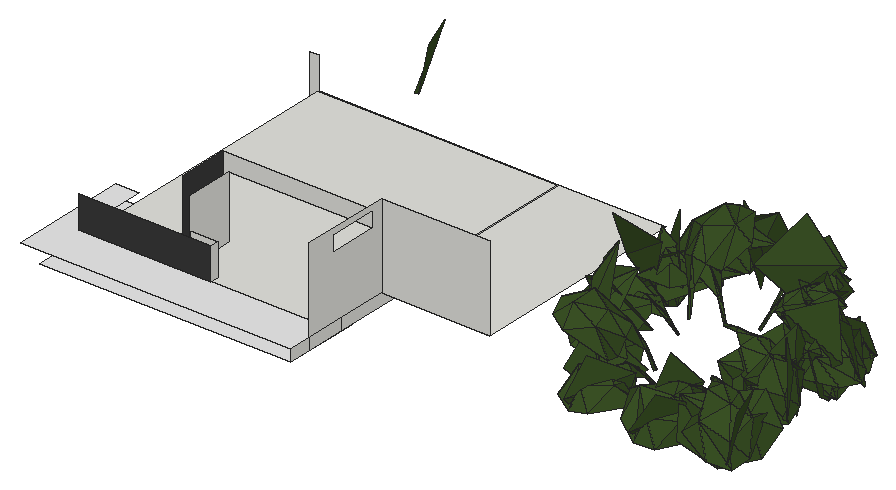
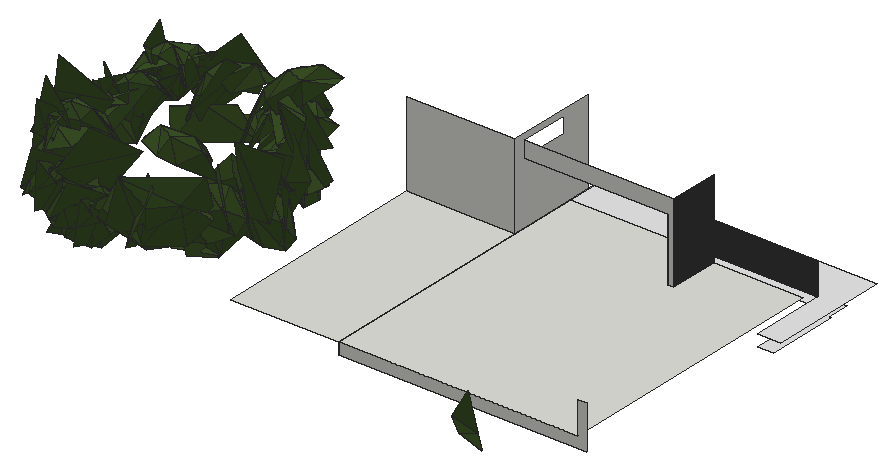
# SketchUp Ruby script. Lengths in inches.
U = 1.inch
M = Sketchup.active_model
def pt(a) = Geom::Point3d.new(a.map { |v| v * U })
def face(e, loops, mat)
  f = e.add_face(loops[0].map { |a| pt(a) })
  loops[1..].each { |l| e.add_face(l.map { |a| pt(a) }).erase! }
  f.material = f.back_material = mat if mat
  f
end
# faces: each face lists its corners as indices into pts; further lists are holes
def faces(e, pts, list, mat = nil) = list.each { |f| face(e, (f[0].is_a?(Array) ? f : [f]).map { |l| l.map { |i| pts[i] } }, mat) }
# xy, xz, yz: faces in a plane at the given z, y or x. An outline is a flat list of corners, or four numbers for a rectangle; further outlines are holes
def ring(l) = l.size == 4 ? [[l[0], l[1]], [l[2], l[1]], [l[2], l[3]], [l[0], l[3]]] : l.each_slice(2).to_a
def flat(e, list, mat, &to3) = list.each { |f| face(e, (f[0].is_a?(Array) ? f : [f]).map { |l| ring(l).map { |u, v| to3.(u, v) } }, mat) }
def xy(e, z, list, mat = nil) = flat(e, list, mat) { |x, y| [x, y, z] }
def xz(e, y, list, mat = nil) = flat(e, list, mat) { |x, z| [x, y, z] }
def yz(e, x, list, mat = nil) = flat(e, list, mat) { |y, z| [x, y, z] }
def lines(e, pts, list) = list.each { |a, b| e.add_line(pt(pts[a]), pt(pts[b])) }
# prism: a flat outline (further loops are holes) pulled along v
def prism(e, loops, v, mat = nil)
  f = face(e, loops, mat); d = Geom::Vector3d.new(v.map { |x| x * U })
  f.pushpull(f.normal.samedirection?(d) ? d.length : -d.length)
end
def box(e, o, s, mat = nil) = prism(e, [[o, [o[0] + s[0], o[1], o[2]], [o[0] + s[0], o[1] + s[1], o[2]], [o[0], o[1] + s[1], o[2]]]], [0, 0, s[2]], mat)
def at(x, y, z, deg = 0) = Geom::Transformation.translation(pt([x, y, z])) * Geom::Transformation.rotation(ORIGIN, Z_AXIS, deg.degrees)
def axes(o, x, y, z) = Geom::Transformation.new([*x, 0, *y, 0, *z, 0, *pt(o).to_a, 1])
def part(name) = M.definitions.add(name)
# library, detail: a bought-in or finely detailed component or shape, given as its bounding box
def library(name, o, s) = part(name).tap { |d| box(d.entities, o, s) }
def detail(e, o, s) = box(e.add_group.entities, o, s)
def put(e, d, t, mat = nil) = e.add_instance(d, t).tap { |i| i.material = mat if mat }
def group(e, t, mat = nil) = e.add_group.tap { |g| g.transformation = t; g.material = mat if mat }.entities
root = M.entities
M.materials.add("AM113_062_Tilia").color = [58, 81, 37]
M.materials.add("[Color M07]").color = [58, 58, 58]
M.materials.add("white_wall").color = [233, 233, 233]
xy(root,500.91,[[413.32,28.625,413.32,82.67,390.32,82.67,390.32,130.3125,385.62,130.3125,385.62,278.26,418.81,278.26,418.81,115.3125,496.21,115.3125,496.21,121.6875,695.48,121.6875,695.48,187.1875,935.92,187.1875,935.92,28.625]],"white_wall")
xy(root,525.1,[[695.48,121.6875,935.92,121.6875,935.92,725.65,436.99,725.65,436.99,139.5,622.42,139.5,622.42,242.3125,635.92,242.3125,635.92,139.5,695.48,139.5],[935.92,265.5,1160.625,725.65]])
xy(root,525.1,[[371.87,28.625,935.92,28.625,935.92,121.6875,418.81,121.6875,418.81,278.26,371.87,278.26]],"white_wall")
xz(root,121.6875,[[418.81,525.1,695.48,592.47]],"[Color M07]")
xz(root,139.5,[[635.92,525.1,695.48,592.47]])
xz(root,242.3125,[[622.42,525.1,622.42,690.29,935.92,690.29,935.92,656.55,635.92,656.55,635.92,525.1]])
xz(root,265.5,[[935.92,525.1,1160.625,701.22]])
xz(root,725.65,[[418.81,500.91,418.81,592.47,436.99,592.47,436.99,525.1,935.92,525.1,935.92,500.91]])
yz(root,622.42,[[139.5,525.1,242.3125,690.29]],"[Color M07]")
yz(root,635.92,[[139.5,525.1,242.3125,656.55]])
yz(root,695.48,[[121.6875,525.1,139.5,592.47]])
yz(root,935.92,[[28.625,500.91,76.875,525.1],[76.875,500.91,160.1875,525.1],[160.1875,500.91,725.65,525.1],[[76.875,525.1,265.5,701.22],[139.5,656.55,242.3125,690.29]]])
p = [[1608.53,201.41,601.09],[1641.49,153.68,545.55],[1685.26,205.85,485.78],[1680.28,206.99,573.08],[1711.38,254.78,570.88],[1727.03,267.14,493.375],
  [1227.45,504.22,507.09],[1257.77,498.2,487.25],[1308.93,432.76,542.29],[1230.67,494.24,489.34],[1237.69,460.03,493.43],[1244.5,488.78,535.27],
  [1286.74,524.49,559.43],[1250.26,531.08,507.09],[1301.88,581.08,490.56],[1299.69,508.34,521.98],[1300.21,541.42,597.74],[1294.36,601.5,579.96],
  [1342.6,650.07,597.52],[1301.32,663.28,529.03],[1620.96,549.03,509.56],[1665.6,554.86,490.94],[1667.41,568.21,523.57],[1682.46,602.0625,491.55],
  [1691.6,430.92,610.26],[1724.02,422.12,539.31],[1691.39,487.72,491.14],[1714.9375,485.36,573.8],[1691.59,538.34,581.77],[1672.27,556.16,507.36],
  [1668.61,633.98,501.61],[1337.11,293.34,491.66],[1387.67,242.25,499.89],[1388.19,266.96,575.1875],[1343.69,304.44,578.2],[1349.98,369.09,590.34],
  [1297.59,350.6,548.22],[1678.86,626.72,509.68],[1656.26,616.84,492.5],[1599.58,597.82,552.56],[1644.91,627.1875,572],[1630.5625,649.05,492.68],
  [1576.24,624.51,514.75],[1745.05,301.41,540.22],[1295.82,401.91,522.83],[1268.66,437.86,545.74],[1511.4,570.35,560.8],[1566.7,592.6875,494.25],
  [1616.57,617.13,543.95],[1503.48,634.35,576.94],[1520.24,677.18,494.31],[1535.15,738.46,525.68],[1599.58,313.53,611.65],[1643.34,292.87,542.47],
  [1654.98,365.88,495.65],[1658.99,353.22,581.5],[1666.94,409.27,590.46],[1667.95,437.21,517.2],[1711.86,395.82,596.52],[1685.69,410.02,495.72],
  [1631.72,447.7,548.77],[1657.73,307.26,600.03],[1661.35,300.36,517.51],[1635.08,376.57,496.53],[1681.1,359.02,557.6],[1677.27,414.18,581.15],
  [1641.67,444.67,526.12],[1453.5,335.59,497.8],[1443.43,306.41,535.73],[1449.4375,309.89,537.47],[1453.22,308.86,531.31],[1456.31,334.82,497.81],
  [1455.86,338.05,501.03],[1301.33,350.89,630.68],[1239.92,360.78,558.58],[1299.97,344.13,498.89],[1367.08,404.5,524.83],[1370.45,429.46,537.58],
  [1276.97,440.16,499.17],[1231.26,429.43,589.95],[1574,282.72,550.39],[1590.74,343.79,499.42],[1458.66,277.01,517.78],[1633.2,294.35,530.68],
  [1427.35,224.91,541.33],[1665.2,614.9375,533.37],[1645.59,642.78,519.97],[1372.92,271.21,623.86],[1333.62,243.31,535.71],[1406.36,250.31,501.97],
  [1433,337.17,524.2],[1543.93,687.91,601.39],[1560.58,714.84,549.01],[1506.53,704.21,502.82],[1508.01,717.95,570.93],[1449.125,701.42,508.87],
  [1462.29,709.39,571.11],[1279.84,345.16,502.99],[1312.67,305.26,522.83],[1304.35,350.98,578.03],[1258.94,412.12,524.86],[1635.5,421.94,588.94],
  [1701.53,411.0625,553.85],[1711.42,482.68,502.96],[1688.85,474.8,584.89],[1680.5,531.22,585.72],[1699.88,555.625,514.64],[1474.65,208.35,538.16],
  [1552.91,206.89,505.11],[1524.41,254.78,555.05],[1614.9375,247.95,507.18],[1286.14,594.98,505.61],[1274.16,520.22,535.21],[1314.23,544.61,597.49],
  [1325.53,603.12,582.9],[1396.83,635.1,561.15],[1329.75,667.15,536.15],[1314.83,358.71,573.32],[1300.05,304.08,539.93],[1359.23,329.29,505.88],
  [1352.78,470.5,565.37],[1301.03,422.38,570.82],[1237.73,477.64,588.08],[1306.48,546.06,533.875],[1662.44,591.39,558.45],[1668.39,175.84,581.64],
  [1696.45,159,523.32],[1731.08,184.67,508.39],[1722.59,190.66,557.13],[1741.22,217.9,518.5],[1417.19,697.9,545.89],[1662.07,319.36,582.11],
  [1688.34,324.3,518.9],[1707.34,363.98,509.22],[1702.21,359.18,558.95],[1703.72,396.45,527.51],[1729.71,172.23,524.3],[1704.85,194.06,509.27],
  [1691.77,269.78,580.98],[569.08,821.01,524.3],[544.22,842.83,509.27],[531.15,918.56,580.98],[1614.36,549.44,538.52],[1602.1,598.66,579.22],
  [1670.43,608.51,577.0625],[1573.15,571.08,602.63],[1611.93,580.5,560.65],[1576.44,619.48,510.05],[1576.88,620.47,580.45],[1536.41,660.93,512.41],
  [1541.04,649.93,575.9],[1720.67,530.4375,617.48],[1728.57,533.34,510.15],[1655.3,557.29,521.91],[1405.16,153.17,541.64],[1411.17,178.17,510.85],
  [1474.36,243.05,547.15],[1492.28,584.64,542.69],[1478.94,575.19,511.11],[1476.91,573.07,513],[1492.97,581.45,547.48],[1479.94,573.09,511.06],
  [1498.32,579.69,547.0625],[1507.43,679.5,545.82],[1322.69,293.23,514.1],[1367.74,234.48,523.55],[1395.16,278.09,571.02],[1363.4,325.46,570.48],
  [1383.97,392.54,535.68],[1315.3,371.51,545.73],[1712.89,350.28,521.46],[1679.92,360.82,514.2],[1644.1,412.73,605.58],[1680.69,590.25,560.28],
  [1513.4,718.2,514.57],[1510.84,695.24,577.86],[1541.9,643.84,579.47],[1564.26,694.65,559.0625],[1465.57,699.29,573.64],[1454.14,722.33,517.46],
  [1589.54,554.74,540.99],[1580.59,544.65,539.82],[1554.89,533.6,519.06],[1556.55,534.56,515.47],[1585.17,544.5,535.56],[1577.37,547.73,537.0625],
  [1555.3125,536.29,516.7],[1674.77,469.17,571.17],[1556.35,651.91,613.09],[1521.76,654.98,517.53],[1502.67,589.41,553.91],[1581.6875,663.6875,534.79],
  [1421.29,711.72,549.26],[1566.69,133.71,524.875],[1598.75,148.19,517.66],[1576.43,153.04,567.01],[1621.69,188.54,559.23],[1646.23,220.55,522.91],
  [1420.59,617.25,621.1],[1401.85,671.68,517.69],[1366.38,742.19,556.95],[1471.69,728.6875,602.9375],[1476.86,740.6,518.39],[1444.36,687.78,518.62],
  [1725.52,246.03,578.39],[1717.69,293.34,564.31],[1483.12,638.75,569.46],[1636.45,304.22,556.29],[1624.37,618.64,560.88],[1585.53,623.89,557.1],
  [1560.79,130.21,545.73],[1556.22,159.39,521.33],[1616.67,228.95,550.25],[1473.58,256.71,521.39],[1468.04,260.58,558.26],[1470.1,204.63,565.96],
  [1506.66,226.96,534.77],[1657.72,416.41,633.88],[1719.05,358.2,610.87],[1611.67,492.47,585.71],[1306.15,475.61,582.13],[1355.55,322.27,560.45],
  [1327.625,433.7,523.27],[1608.23,245.3,529.97],[1639.7,168.85,555.37],[1323.03,438.05,559.67],[1381.29,222.1,568.35],[1377.32,174.28,531.56],
  [1415.8,152.53,523.625],[1419.43,176.86,562.98],[1450.18,161.58,526.36],[1412.87,219.85,554.3],[1634.27,587.6,560],[1412.17,553.15,566.37],
  [1438.04,536.35,527.79],[1435.375,538.43,523.96],[1408.89,559.38,562.98],[1704.6,272.01,610.13],[1735.45,191.29,610.92],[543.97,920.79,610.13],
  [574.82,840.0625,610.92],[1536.19,189.6,597.59],[1529.56,147.08,551.74],[1284.17,401.26,605.55],[1321.77,452.63,626.16],[1261.18,466.59,604.29],
  [1410.2,548.1875,561.41],[1434.3125,535.63,525.01],[1499.07,721.84,601.54],[1542.79,546.8,567.91],[1597.85,563.92,564.49],[1589.35,621.96,526.02],
  [1560.88,603.25,580.4375],[1535.32,640.78,575.46],[1553.72,669.54,527.3125],[1658.55,474.5,579.81],[1519.73,684.8125,553.46],[1684.07,406.65,594.57],
  [1655.95,447.01,594.14],[1366.85,686.33,528.33],[1314.39,637.14,535.91],[1320.47,655.41,613.81],[1357.14,700.64,613.59],[1415.74,701.12,651.71],
  [1409.78,740.29,586.14],[1403.52,274,528.53],[1359.78,234.46,534.93],[1422.1,280.59,556.48],[1611.18,243.47,567.59],[1461.57,265.78,530.04],
  [1280.85,564.23,638.51],[1253.03,552.57,530.6],[1318.49,502.35,533.64],[1445.99,273.75,571.29],[1374.88,451.56,553.33],[1406.8,448.44,531.47],
  [1409.12,448.6875,535.73],[1263.05,341.63,531.83],[1250.26,413.28,551.72],[1557.84,196.35,585.28],[1554.79,207.85,542.72],[1564.06,301.86,531.88],
  [1566.56,316.89,559.1875],[1374.54,455.09,559.72],[1407.6,451.18,531.9],[1371.82,461.16,557.1],[1395.05,556.37,572.13],[1756.79,484.03,559.74],
  [1728.09,485.14,533.77],[1654.7,529.06,586.64],[1343.99,501.77,540.33],[1585.03,291.13,560.35],[1576.95,321.07,534.7],[1576.89,323.73,538.73],
  [1587.31,591.74,534.94],[1597.89,582.3,559.06],[1289.01,483.91,587.59],[1288.87,466.49,571.02],[1607.62,562.51,559.41],[1574.2,321.33,535.88],
  [1577.11,286.48,567.33],[1582.77,290.6875,567.76],[1286.8,607.89,582.24],[1449.44,311.51,578.55],[1455.06,326.86,535.96],[1457.43,329.96,537.64],
  [1479.73,626.03,562.03],[1477.46,604.47,536.34],[1477.82,601.97,539.04],[1482.75,625.38,567.01],[1479.71,603.87,536.36],[1487.54,628.14,565.49],
  [1453.36,329.1875,536.52],[1442.17,316,586.78],[1449.05,315.19,584.94],[1300.2,386.02,635.55],[1603.91,476.61,631.84],[1671.75,470.05,539.75],
  [1744.25,456.05,593.02],[1689.67,325.37,584.79],[1388.31,501.26,584.9],[1396.27,491.48,540.24],[1397.25,487.57,541.29],[1343.37,482.55,568.05],
  [1517.42,750.8,564.1],[1512.8,730.06,540.52],[1462.52,678.86,571.92],[1391.52,498.69,590.85],[1399.16,491.32,540.72],[1396.44,503.38,593.35],
  [1448.09,263.88,582.71],[1251.37,617.26,574.06],[1274.45,602.33,541.53],[1340.4,536.98,592.33],[1484.12,242.45,578.33],[1429.1,183.04,617.29],
  [1343.82,317.33,542.08],[1368.51,275.21,571.57],[1334.83,311.12,622.63],[1310.1,379.3125,561.62],[1512.48,595.88,581.375],[1510.26,616.82,572.9],
  [1377.64,602.7,546.0625],[1340.45,653.39,542.68],[1328.47,639.1,585.61],[1275.19,641.54,552.01],[1698.77,443.05,593.95],[1741.88,452.39,549.85],
  [1753.04,495.28,543.03],[1732.9,491.17,586.0625],[1736.62,526.27,550.97],[1362.07,705.24,543.05],[1302.21,661.14,546.67],[1331.8,648.4375,616.98],
  [1378.25,681.28,622.25],[1449.53,657.45,624.27],[1429.66,724.02,598.73],[1569.18,626.8125,610.93],[1513.68,624.38,544.59],[1541.48,646.34,590.125],
  [1512.69,658.9375,559.67],[1633.29,226.17,575.92],[1597.59,153.94,616.24],[1334.71,498.53,658.14],[1295.15,522.89,545.81],[1218.48,552.85,571.01],
  [1493.91,653.65,587.63],[1429.37,679.14,594.18],[1464.0625,575.04,628.03],[1508.4,636.16,546.03],[1556.66,685.63,608.96],[1385.41,588.23,580.21],
  [1279.5,624.4,586.46],[1522.42,578.75,569.41],[1479.8125,646.38,548.27],[1596.48,387.05,626.5],[1424.73,656.99,560.77],[1565.26,488.62,549.54],
  [1599.68,484.26,581.49],[1595.12,489.16,584.42],[1562.68,490.16,553.375],[1538.97,572.53,549.625],[1584.35,565.88,564.44],[1576.9,583.29,592.19],
  [1508.96,750.82,549.65],[1506.09,732.35,582.05],[1536.74,696.53,588.3125],[1539.78,733.82,557],[1481.52,743.51,552.09],[1688.36,420.6875,560.36],
  [1594.58,493.35,578.59],[1565.35,491.52,549.75],[1694.67,533.41,598.9375],[1661.38,564.78,575.59],[1506.51,202.02,577.12],[1309.6,413.16,594.18],
  [1285.73,478.125,598.61],[1463.26,667.33,551.92],[1467.625,665.17,581.53],[1465.71,710.01,585.4],[1436.67,691.26,561.28],[1248.15,602.93,559.16],
  [1333,458.92,578.08],[1627.39,225.02,573.375],[1603.92,346.24,589.86],[1439.68,229.05,581.32],[1345.46,697.09,651.89],[1554.06,685.94,562.21],
  [1694.47,227.08,602.17],[1647.74,567.875,619.08],[1504.42,649.36,581.08],[1519.3,654.02,558.56],[1666.41,373.3,614.51],[1593.59,204.98,590.92],
  [1547.15,254.95,632.8],[1254.87,567.09,572.36],[1276.94,604.01,598],[1656.28,537.29,618.49],[1730.39,496.66,641.81],[1581.57,658.72,568.625],
  [1616.39,569.27,581.08],[1591.8125,250.76,591.14],[1639.4375,453.77,564.95],[1362.92,482.23,589.49],[1377.4,567.29,604.16],[1360.41,543.62,599.62],
  [1301.33,355.875,643.62],[1319.89,402.95,697.53],[1275.04,419.93,642.01],[1485.27,655.07,592.54],[1639.03,526.12,563.15],[1640.46,518.2,599.58],
  [1301.97,549.33,614.71],[1319.48,503.23,592.21],[1352.57,531.28,564.02],[1454.65,680.0625,596.76],[1498.26,728.69,625.63],[1674.04,279.89,564.21],
  [1677.1,269.65,599.5],[1611.25,607.63,573.1875],[1631.7,468.9375,595.7],[1541.59,248.89,566.1],[1564.92,255.05,587.52],[1584.5,630,595.51],
  [1605.04,642.65,569.75],[1541.13,614.41,598.5],[1223.35,508.6,670.14],[1619.55,460.53,624.52],[1388.68,285.97,635.5],[1637.89,238.61,603.98],
  [1341.65,533.01,627.7],[1287.41,603.79,656.33],[1437.88,292.14,632.31],[1443.43,267.15,618.99],[1634.27,493.08,611.99],[1658.56,447.66,641.11],
  [1331.75,580.78,617.54],[1624.02,282.6,597.95],[1596.29,302.82,580.66],[1594.22,303.2,585.21],[1594.28,300.72,580.79],[1622.29,272.2,599.91],
  [1622.82,278.57,603.8],[1490.09,691.04,598.75],[1610.88,358.78,622.8125],[1339.49,499.76,634.89],[1313.61,599.875,642.68],[1381.02,517.07,641.75],
  [1357.82,529.38,630.81],[1417.86,222.85,649.35],[1447.39,215.08,599.6],[1434.125,257.37,585.35],[1679.85,497.35,614.41],[1327.14,575,600.87],
  [1418.98,310.76,623.63],[1622.22,416.21,593.02],[1632.85,403.82,624.51],[1706.75,490.57,686.85],[1407.24,521.16,633.07],[1658.74,253.62,616.19],
  [1367.96,197.78,638.26],[1355.49,545.84,599.58],[1339.4,573.66,668.86],[1314.31,560.16,617.14],[1392.92,314.4375,607.04],[1341.25,310.9,643.96],
  [1361.21,291.11,672.7],[1504.49,664.71,697.67],[1624.68,379.48,637.56],[1350.62,629,666.25],[1412.68,261.97,662.65],[1428.375,573.59,690.4],
  [1426.09,540.78,619.0625],[1455.9,579.69,661.8],[1543.48,397.94,619.66],[1582.49,382.3,628.9],[1580.73,387.65,634.39],[1542.85,399.53,624.66],
  [1579.53,392.52,629.71],[1544.41,400.7,619.99],[1373.44,552.375,678.12],[1336.56,211.51,650.76],[1364.29,231.9,674.93],[1321.63,252.8,661.06],
  [1422.81,629.08,687.64],[1380.11,607.39,699.11],[1381.05,643.83,680.53]]
faces(root,p,[[0,1,2],[2,3,0],[4,3,2],[2,5,4],[6,7,8],[9,10,11],[9,11,12],[12,13,9],
  [14,15,16],[16,17,14],[14,17,18],[18,19,14],[20,21,22],[22,21,23],[24,25,26],[26,27,24],
  [28,27,26],[26,29,28],[22,23,30],[31,32,33],[33,34,31],[35,36,31],[31,34,35],[37,38,39],
  [40,41,42],[5,43,4],[10,44,45],[11,10,45],[46,47,48],[49,50,51],[52,53,54],[54,55,52],
  [56,55,54],[54,57,56],[58,59,60],[61,62,63],[63,64,61],[65,64,63],[63,66,65],[67,68,69],
  [70,71,72],[69,72,67],[73,74,75],[73,75,76],[77,78,79],[80,81,82],[80,83,81],[32,84,33],
  [72,69,70],[30,85,22],[30,86,85],[87,88,89],[87,89,90],[91,92,93],[93,94,91],[93,95,96],
  [96,94,93],[97,98,99],[100,97,99],[101,102,103],[103,104,101],[105,104,103],[103,106,105],[82,107,108],
  [108,109,82],[80,109,108],[108,110,80],[111,112,113],[113,114,111],[115,116,111],[111,114,115],[117,118,119],
  [117,119,120],[8,121,6],[121,122,6],[12,123,13],[110,83,80],[29,124,28],[125,126,127],[127,128,125],
  [127,129,128],[95,130,96],[131,132,133],[133,134,131],[133,135,134],[136,137,138],[139,140,141],[22,142,20],
  [39,143,37],[143,144,37],[145,146,147],[147,148,145],[147,149,150],[150,148,147],[151,152,153],[154,155,156],
  [157,158,159],[160,159,161],[161,162,160],[149,163,150],[159,160,157],[164,165,166],[166,167,164],[168,169,164],
  [164,167,168],[170,171,172],[106,173,105],[174,175,176],[176,177,174],[178,175,174],[174,179,178],[40,42,180],
  [181,182,183],[183,184,181],[185,186,182],[57,187,56],[188,189,190],[188,191,189],[179,192,178],[193,194,195],
  [195,194,196],[194,197,196],[198,199,200],[82,109,80],[201,202,203],[128,129,204],[129,205,204],[201,203,206],
  [131,207,132],[182,181,185],[85,86,208],[86,209,208],[210,211,212],[213,214,215],[215,216,213],[172,217,170],
  [217,218,170],[151,153,219],[15,220,16],[99,98,221],[45,44,222],[196,197,223],[125,224,126],[222,225,45],
  [226,227,228],[228,229,226],[228,230,229],[165,231,166],[142,22,232],[22,85,232],[233,234,235],[235,236,233],
  [138,237,136],[237,238,136],[141,239,139],[239,240,139],[241,242,193],[193,195,241],[99,243,100],[100,243,244],
  [244,245,100],[246,247,234],[248,49,51],[249,250,251],[251,252,249],[253,252,251],[251,254,253],[66,255,65],
  [229,230,215],[230,216,215],[254,256,253],[134,135,257],[135,258,257],[234,233,246],[259,260,261],[261,262,259],
  [259,262,263],[263,264,259],[265,266,226],[226,267,265],[223,268,196],[166,231,269],[166,269,168],[270,271,272],
  [273,214,70],[70,69,273],[274,275,276],[226,266,227],[277,118,117],[278,277,117],[279,280,281],[281,282,279],
  [283,276,284],[284,285,283],[232,85,208],[270,272,286],[287,288,289],[290,123,12],[291,292,293],[294,295,208],
  [208,209,294],[112,296,113],[297,11,45],[12,11,297],[298,181,184],[184,142,298],[68,267,273],[273,69,68],
  [168,167,166],[276,283,274],[299,300,301],[301,293,299],[260,302,261],[303,304,305],[306,307,308],[309,308,310],
  [310,311,309],[312,313,314],[314,305,312],[185,181,298],[298,295,185],[305,314,303],[315,77,79],[232,298,142],
  [293,301,291],[308,309,306],[316,317,318],[4,43,319],[320,321,322],[12,323,290],[324,325,326],[327,322,328],
  [328,329,327],[33,84,330],[322,327,320],[331,332,333],[156,334,154],[334,335,154],[336,337,338],[339,336,338],
  [157,160,340],[340,341,157],[342,343,344],[344,343,345],[346,347,348],[348,349,346],[348,350,349],[351,352,353],
  [353,354,351],[355,356,351],[351,354,355],[357,46,48],[358,341,359],[359,360,358],[212,361,210],[361,362,210],
  [297,45,225],[363,364,365],[150,163,366],[96,130,367],[368,369,370],[344,371,342],[352,372,353],[162,373,340],
  [340,160,162],[253,374,249],[253,256,374],[58,60,375],[178,192,376],[377,378,379],[379,380,377],[381,382,383],
  [383,373,381],[384,385,386],[386,387,384],[384,388,385],[346,389,347],[390,391,380],[349,350,392],[350,393,392],
  [241,394,242],[117,395,278],[278,395,120],[120,396,278],[397,398,399],[399,400,397],[344,345,401],[388,400,399],
  [385,388,399],[402,225,274],[274,283,402],[380,379,390],[403,224,125],[404,207,131],[267,226,405],[405,273,267],
  [406,198,200],[386,407,387],[125,128,408],[408,128,204],[402,283,285],[285,323,402],[61,64,65],[405,215,214],
  [405,214,273],[28,124,409],[386,410,411],[411,407,386],[131,134,412],[412,134,257],[232,295,298],[232,208,295],
  [413,195,196],[413,196,268],[282,414,279],[401,415,416],[401,416,344],[323,12,297],[297,225,402],[289,417,287],
  [417,418,287],[419,360,359],[105,173,420],[421,268,291],[291,301,421],[99,221,244],[422,389,346],[178,376,176],
  [113,423,115],[115,114,113],[424,425,246],[246,233,424],[338,426,339],[339,426,427],[427,428,339],[306,309,429],
  [429,398,306],[226,229,405],[405,229,215],[424,233,236],[236,371,424],[430,431,392],[392,393,430],[432,433,434],
  [434,425,432],[326,435,324],[435,436,324],[204,205,437],[437,438,204],[383,382,439],[346,440,422],[120,395,117],
  [429,309,311],[311,410,429],[441,394,241],[241,442,441],[241,195,413],[300,442,421],[421,301,300],[413,268,421],
  [249,252,253],[297,402,323],[443,419,359],[444,419,443],[445,340,373],[373,383,445],[383,439,444],[444,443,383],
  [4,319,0],[0,3,4],[91,94,96],[446,363,365],[96,367,91],[56,187,447],[338,337,448],[415,433,432],
  [416,415,432],[445,341,340],[445,359,341],[125,449,403],[176,175,178],[24,27,28],[333,450,331],[450,451,331],
  [33,330,35],[35,34,33],[150,366,145],[145,148,150],[244,243,99],[408,204,438],[452,453,303],[303,314,452],
  [390,379,454],[454,431,390],[65,255,455],[18,17,16],[456,424,371],[371,344,456],[457,458,459],[460,461,462],
  [462,459,460],[105,420,101],[463,429,410],[410,386,463],[65,455,61],[52,55,56],[378,440,454],[454,379,378],
  [463,398,429],[463,399,398],[449,125,408],[28,409,24],[131,464,404],[464,131,412],[16,220,465],[463,385,399],
  [386,385,463],[261,302,466],[452,314,313],[101,104,105],[320,327,467],[467,468,320],[459,462,457],[469,470,471],
  [471,453,469],[344,416,456],[346,349,472],[472,349,392],[353,372,473],[313,474,452],[442,241,413],[413,421,442],
  [113,296,423],[445,443,359],[56,447,52],[467,327,329],[383,443,445],[475,476,257],[257,258,475],[477,316,318],
  [329,478,467],[440,346,472],[412,257,476],[472,454,440],[16,465,18],[457,462,479],[479,438,457],[456,416,432],
  [472,392,431],[408,438,479],[480,470,469],[472,431,454],[481,468,482],[456,432,425],[456,425,424],[482,483,481],
  [461,449,479],[479,462,461],[353,473,355],[408,479,449],[484,485,486],[486,474,484],[487,368,370],[263,262,261],
  [261,466,263],[412,488,464],[412,476,488],[355,354,353],[489,483,482],[490,469,453],[490,453,452],[491,478,492],
  [492,493,491],[494,495,496],[496,497,494],[498,499,497],[338,448,427],[427,426,338],[495,464,488],[474,486,490],
  [490,452,474],[488,476,498],[497,496,498],[488,496,495],[498,496,488],[500,468,467],[500,482,468],[500,467,478],
  [478,491,500],[501,480,502],[502,480,469],[486,485,503],[490,502,469],[486,503,501],[501,502,486],[491,493,504],
  [486,502,490],[505,489,482],[506,489,505],[500,505,482],[491,505,500],[506,505,491],[491,504,506]],"AM113_062_Tilia")
